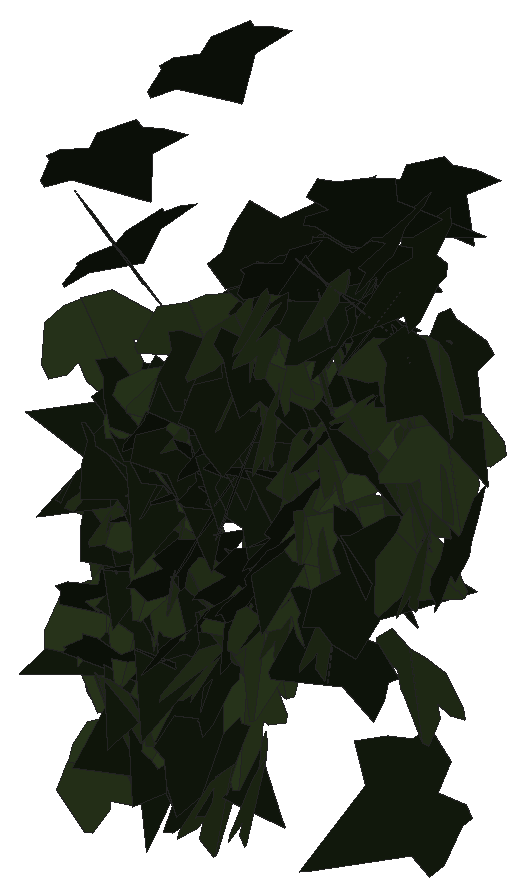
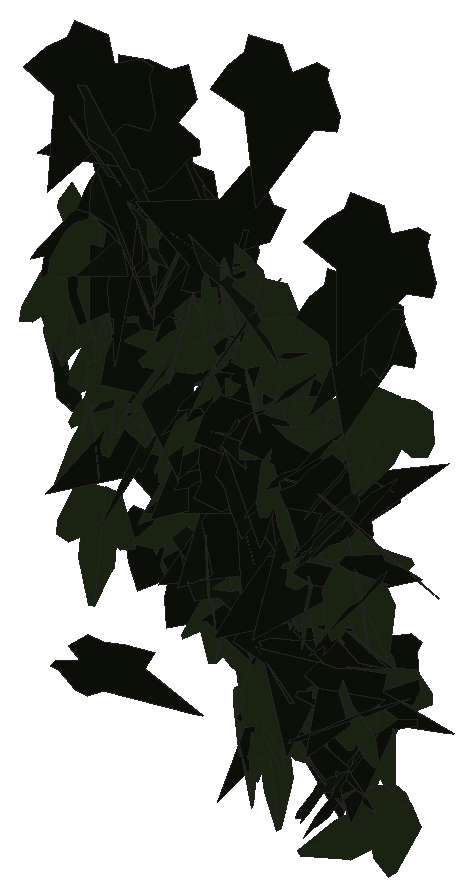
# SketchUp Ruby script. Lengths in inches.
U = 1.inch
M = Sketchup.active_model
def pt(a) = Geom::Point3d.new(a.map { |v| v * U })
def face(e, loops, mat)
  f = e.add_face(loops[0].map { |a| pt(a) })
  loops[1..].each { |l| e.add_face(l.map { |a| pt(a) }).erase! }
  f.material = f.back_material = mat if mat
  f
end
# faces: each face lists its corners as indices into pts; further lists are holes
def faces(e, pts, list, mat = nil) = list.each { |f| face(e, (f[0].is_a?(Array) ? f : [f]).map { |l| l.map { |i| pts[i] } }, mat) }
# xy, xz, yz: faces in a plane at the given z, y or x. An outline is a flat list of corners, or four numbers for a rectangle; further outlines are holes
def ring(l) = l.size == 4 ? [[l[0], l[1]], [l[2], l[1]], [l[2], l[3]], [l[0], l[3]]] : l.each_slice(2).to_a
def flat(e, list, mat, &to3) = list.each { |f| face(e, (f[0].is_a?(Array) ? f : [f]).map { |l| ring(l).map { |u, v| to3.(u, v) } }, mat) }
def xy(e, z, list, mat = nil) = flat(e, list, mat) { |x, y| [x, y, z] }
def xz(e, y, list, mat = nil) = flat(e, list, mat) { |x, z| [x, y, z] }
def yz(e, x, list, mat = nil) = flat(e, list, mat) { |y, z| [x, y, z] }
def lines(e, pts, list) = list.each { |a, b| e.add_line(pt(pts[a]), pt(pts[b])) }
# prism: a flat outline (further loops are holes) pulled along v
def prism(e, loops, v, mat = nil)
  f = face(e, loops, mat); d = Geom::Vector3d.new(v.map { |x| x * U })
  f.pushpull(f.normal.samedirection?(d) ? d.length : -d.length)
end
def box(e, o, s, mat = nil) = prism(e, [[o, [o[0] + s[0], o[1], o[2]], [o[0] + s[0], o[1] + s[1], o[2]], [o[0], o[1] + s[1], o[2]]]], [0, 0, s[2]], mat)
def at(x, y, z, deg = 0) = Geom::Transformation.translation(pt([x, y, z])) * Geom::Transformation.rotation(ORIGIN, Z_AXIS, deg.degrees)
def axes(o, x, y, z) = Geom::Transformation.new([*x, 0, *y, 0, *z, 0, *pt(o).to_a, 1])
def part(name) = M.definitions.add(name)
# library, detail: a bought-in or finely detailed component or shape, given as its bounding box
def library(name, o, s) = part(name).tap { |d| box(d.entities, o, s) }
def detail(e, o, s) = box(e.add_group.entities, o, s)
def put(e, d, t, mat = nil) = e.add_instance(d, t).tap { |i| i.material = mat if mat }
def group(e, t, mat = nil) = e.add_group.tap { |g| g.transformation = t; g.material = mat if mat }.entities
root = M.entities
M.materials.add("efeu1").color = [18, 25, 13]
M.materials.add("efeu2").color = [43, 57, 29]
c1 = part("ivyleaf_10")
p = [[0,0.5,-0.03],[-0.0625,2.02,-0.43],[-0.19,2.01,-0.46],[-0.54,1.05,-0.29],[-0.52,0.625,-0.18],[-0.83,0.76,-0.28],
  [-1.16,0.64,-0.33],[-1.15,0.33,-0.24],[-0.77,-0.39,0.02],[-0.3,-0.51,0.16],[0.04,-0.48,0.23],[-0.02,2.01,-0.4375],
  [-0.06,2.01,-0.43],[0.04,-0.49,0.23],[0.67,-0.49,0.14],[1.38,0.36,-0.2],[1.375,0.51,-0.24],[0.81,0.65,-0.19],
  [0.62,0.59,-0.15],[0.6,1.09,-0.28],[0.5,1.23,-0.31]]
faces(c1.entities,p,[[0,1,2,3,4,5,6,7,8,9,10],[11,12,0,13,14,15,16,17,18,19,20]],"efeu2")
c2 = part("ivyleaf_9")
p = [[1.54,2.16,1.25],[1.36,2.04,1.19],[-0.21,0.99,0.68],[-0.71,1.11,0.82],[-0.85,0.86,0.67],[-0.8,0.17,0.21],
  [-0.9,-0.01,0.1],[-0.67,-0.16,-0.02],[-0.08,-0.08,-0.05],[-0.03,-0.6,-0.4],[0.65,-0.88,-0.66],[0.83,-0.6,-0.49],
  [1.29,-0.42,-0.43],[1.8125,-0.07,-0.26],[1.21,0.44,0.15]]
faces(c2.entities,p,[[0,1,2,3,4,5,6,7,8,9,10,11,12,13,14]],"efeu1")
put(root,c1,axes([35.52,223.96,228.77],[-0.15794,-0.42054,-0.21955],[0.07489,0.20639,-0.44921],[0.46845,-0.17478,-0.0022]))
put(root,c1,axes([35.24,224.09,223.65],[0.05182,-0.4899,-0.0855],[-0.02172,0.08365,-0.49247],[0.49683,0.05475,-0.01262]))
put(root,c2,axes([37,223.73,226.66],[0.10287,0.0619,-0.48537],[-0.07928,0.49154,0.04589],[0.48284,0.06752,0.11094]))
put(root,c1,axes([35.87,224.14,228.92],[0.06062,-0.49536,-0.03074],[0.00028,0.03101,-0.49904],[0.49631,0.06048,0.00404]))
put(root,c1,axes([34.51,224.03,227.63],[0.41045,0.27365,0.08151],[0.02159,0.11258,-0.48668],[-0.28472,0.40304,0.0806]))
put(root,c1,axes([35.71,224.14,229.06],[0.16315,-0.47129,-0.03561],[0.00214,0.03841,-0.49852],[0.47263,0.16252,0.01455]))
put(root,c1,axes([34.15,224.17,225.34],[0.49772,-0.0464,-0.01106],[-0.01119,-0.0008,-0.49987],[0.04637,0.49784,-0.00183]))
put(root,c2,axes([35.02,224.33,227.81],[-0.03439,-0.49861,-0.01448],[0.00897,0.0139,-0.49973],[0.49874,-0.03463,0.00799]))
put(root,c1,axes([37.9,224.14,228.24],[-0.26587,-0.42079,-0.04744],[0.13104,-0.02848,-0.48168],[0.40267,-0.26856,0.12542]))
put(root,c1,axes([33.87,224.05,224.1],[-0.45825,0.19556,-0.04199],[0.03608,-0.02242,-0.49819],[-0.19673,-0.45962,0.00644]))
put(root,c2,axes([34.05,224.23,227.47],[0.25315,-0.43099,0.01288],[0.02635,0.00056,-0.49931],[0.43037,0.25348,0.02299]))
put(root,c1,axes([37.78,224.09,229.05],[0.4487,-0.2169,0.04034],[0.10045,0.11946,-0.47501],[0.19642,0.43438,0.15078]))
put(root,c2,axes([35.21,223.92,223.78],[-0.24544,0.33182,0.28223],[-0.19825,0.20337,-0.41151],[-0.38789,-0.31391,0.03174]))
put(root,c1,axes([37.67,224.04,227.08],[0.19131,-0.42538,-0.18014],[-0.04582,0.17654,-0.46555],[0.45968,0.19463,0.02857]))
put(root,c1,axes([36.54,224.09,226],[0.14851,-0.46443,-0.11067],[0.00063,0.11609,-0.48634],[0.47744,0.14431,0.03506]))
put(root,c2,axes([36.74,224.11,225.74],[0.06549,0.0969,-0.48613],[-0.41934,-0.25065,-0.10645],[-0.26433,0.42165,0.04844]))
put(root,c1,axes([35.8125,224.09,227.92],[0.22839,-0.43074,-0.11089],[0.01971,0.13434,-0.48121],[0.44435,0.21544,0.07835]))
put(root,c2,axes([33.77,223.99,229.26],[0.46569,-0.11467,-0.14136],[-0.13181,0.05537,-0.47913],[0.12554,0.48351,0.02134]))
put(root,c2,axes([36.75,223.875,230.49],[0.38317,0.08091,0.31086],[0.2953,0.10168,-0.39046],[-0.1264,0.48282,0.03014]))
put(root,c2,axes([35.46,223.85,228.18],[0.15851,-0.12531,-0.45735],[-0.07051,0.47064,-0.15339],[0.46894,0.11312,0.13153]))
put(root,c2,axes([34.33,224.38,226.8125],[-0.14137,-0.00782,0.47954],[-0.44716,-0.17859,-0.13473],[0.17339,-0.46695,0.0435]))
put(root,c2,axes([35.56,223.77,226.95],[0.08008,0.07508,0.4878],[0.04245,0.4913,-0.08258],[-0.49172,0.05464,0.07231]))
put(root,c2,axes([35.19,224.24,228.19],[-0.17493,-0.40483,-0.23561],[0.09349,0.21627,-0.44101],[0.45898,-0.19835,0.00003]))
put(root,c2,axes([36.64,224.09,229.3125],[-0.32127,0.28919,0.25131],[-0.27364,0.05635,-0.41466],[-0.26815,-0.40397,0.12206]))
put(root,c2,axes([35.75,224.41,226.88],[-0.10894,-0.4873,0.02594],[-0.00635,-0.02516,-0.49933],[0.48795,-0.10913,-0.00071]))
put(root,c2,axes([37.68,224.18,230.17],[-0.44218,0.23119,-0.0321],[0.02923,-0.01336,-0.49897],[-0.23157,-0.44314,-0.0017]))
put(root,c1,axes([36.25,224.19,229.26],[-0.44111,-0.17762,0.15452],[-0.12742,-0.09582,-0.4739],[0.19796,-0.45746,0.03927]))
put(root,c1,axes([35.34,224.23,228.03],[0.23101,-0.44309,0.0175],[0.00756,-0.0158,-0.49969],[0.44337,0.23113,-0.0006]))
put(root,c2,axes([36.02,224.14,229.07],[0.2194,-0.08043,0.44203],[0.41564,-0.15045,-0.23368],[0.17059,0.47,0.00084]))
put(root,c1,axes([34.9,224.11,228.55],[-0.39357,-0.27685,-0.13587],[0.14092,0.0345,-0.47849],[0.27431,-0.41493,0.05087]))
put(root,c2,axes([34.125,224.54,223.59],[-0.06005,-0.32774,0.3728],[0.07015,-0.37735,-0.32044],[0.4914,0.01382,0.09131]))
put(root,c2,axes([35.14,223.88,231.61],[0.17246,0.4691,0.01434],[0.00467,0.01356,-0.49979],[-0.46929,0.17252,0.0003]))
put(root,c1,axes([34.29,224.23,225.95],[-0.36066,-0.22563,0.26271],[-0.22969,-0.12801,-0.42527],[0.25916,-0.42744,-0.01132]))
put(root,c2,axes([34.5,224.39,227.09],[-0.32415,-0.37301,-0.07607],[0.05769,0.05063,-0.49407],[0.37629,-0.32909,0.01022]))
put(root,c1,axes([35.59,224.13,223.83],[0.19074,-0.44344,-0.13031],[-0.03973,0.12472,-0.48256],[0.46048,0.19444,0.01234]))
put(root,c2,axes([35.52,224.0625,228.62],[0.29268,-0.3076,-0.26405],[-0.1591,0.21238,-0.42377],[0.37286,0.33208,0.02644]))
put(root,c2,axes([36.17,223.875,229.68],[0.31164,0.39051,0.01944],[0.00341,0.02214,-0.4995],[-0.39098,0.31146,0.01113]))
put(root,c2,axes([34.07,223.99,224.62],[0.32074,0.2814,-0.26065],[-0.24394,-0.11256,-0.42169],[-0.29601,0.39767,0.06509]))
put(root,c2,axes([33.95,224.57,223.63],[0.20155,-0.28904,-0.35474],[0.19057,-0.29938,0.35221],[-0.41601,-0.27718,-0.01051]))
put(root,c2,axes([34.23,224.26,226.83],[-0.47418,0.14861,0.05541],[-0.06972,-0.03843,-0.49362],[-0.14246,-0.47585,0.05717]))
put(root,c2,axes([33.8,223.88,230.11],[0.26621,0.42299,0.0144],[0.00483,0.01397,-0.49978],[-0.42321,0.26624,0.00336]))
put(root,c1,axes([34.875,224.16,225.67],[-0.42422,0.13348,-0.22852],[0.21515,-0.07748,-0.44464],[-0.15412,-0.47558,0.0083]))
put(root,c1,axes([33.64,224.03,228.09],[0.36696,0.27323,0.20171],[0.08739,0.21099,-0.4448],[-0.32818,0.3617,0.1071]))
put(root,c1,axes([36.57,224.21,229.46],[0.08804,-0.49081,-0.0368],[-0.00027,0.03734,-0.4986],[0.49219,0.08782,0.00631]))
put(root,c1,axes([34.82,224.24,227.69],[-0.35532,-0.35131,0.01808],[0.05364,-0.0795,-0.49072],[0.34767,-0.34678,0.09418]))
put(root,c2,axes([36.77,224.1,229.31],[-0.34402,0.36065,0.03972],[-0.0341,0.02235,-0.49833],[-0.36123,-0.34559,0.00922]))
put(root,c2,axes([35.45,224.33,228.05],[-0.06953,-0.46957,-0.15707],[0.04009,0.15275,-0.4744],[0.49352,-0.07856,0.01641]))
put(root,c2,axes([37.27,223.98,229.53],[-0.17331,0.46218,0.07969],[-0.01226,0.08046,-0.49333],[-0.46884,-0.17295,-0.01655]))
put(root,c2,axes([35.02,224.02,224.22],[0.13723,-0.27077,-0.3973],[-0.13808,0.37357,-0.30229],[0.46054,0.19269,0.02776]))
put(root,c2,axes([33.99,224.28,226.86],[0.09239,-0.4653,-0.15799],[-0.01471,0.15806,-0.47413],[0.49117,0.09225,0.01552]))
put(root,c2,axes([34.63,224.38,227.22],[0.04884,-0.49538,-0.04705],[-0.00109,0.04717,-0.49777],[0.49761,0.04873,0.00353]))
put(root,c2,axes([37.65,224.19,229.17],[0.12942,-0.41312,-0.25017],[-0.06756,0.24096,-0.43287],[0.47821,0.14584,0.00654]))
put(root,c1,axes([35.68,224.1875,228.48],[0.49581,-0.06398,0.00868],[0.02156,0.10071,-0.48928],[0.06086,0.48556,0.10262]))
put(root,c1,axes([37.56,224.18,227.91],[-0.43961,0.21485,0.10286],[-0.14183,-0.06262,-0.47536],[-0.19138,-0.44712,0.116]))
put(root,c1,axes([35.24,224.46,226.33],[0.06548,-0.06117,0.4919],[0.41809,-0.25974,-0.08796],[0.26629,0.42284,0.01713]))
put(root,c2,axes([35.78,223.8,226.12],[0.13919,0.35786,0.32026],[0.08866,0.30855,-0.38332],[-0.47198,0.1635,0.02244]))
put(root,c1,axes([34.4,224.5,225.96],[-0.12843,0.20564,-0.43729],[0.11586,-0.42617,-0.23443],[-0.46913,-0.16155,0.06181]))
put(root,c1,axes([34.82,224.27,227.46],[0.46548,0.17948,-0.03337],[-0.02644,-0.02414,-0.49872],[-0.18063,0.46605,-0.01298]))
put(root,c2,axes([36.81,224.09,229.92],[0.29238,0.33013,-0.23564],[-0.16206,-0.17121,-0.44094],[-0.37182,0.33422,0.00688]))
put(root,c2,axes([36.06,223.81,226.73],[0.12825,0.32142,0.36089],[0.11646,0.34182,-0.34582],[-0.46903,0.17276,0.01282]))
put(root,c1,axes([37.38,224.22,228.95],[-0.41138,-0.28403,-0.0096],[0.01363,-0.00286,-0.49981],[0.28387,-0.41148,0.0101]))
put(root,c2,axes([34.5,224.49,225.22],[-0.28829,-0.40651,-0.04048],[0.04771,0.01571,-0.49747],[0.40573,-0.29069,0.02973]))
put(root,c1,axes([34.39,224.32,226.09],[0.31111,0.35743,-0.15954],[-0.10617,-0.1191,-0.47386],[-0.37675,0.32872,0.00179]))
put(root,c2,axes([34.05,223.92,229.15],[0.09935,0.4815,0.09101],[-0.03175,0.099,-0.48907],[-0.489,0.0914,0.05025]))
put(root,c2,axes([37.41,224.07,230.44],[-0.25608,0.42072,0.08615],[-0.05093,0.06985,-0.49247],[-0.42642,-0.261,0.00708]))
put(root,c2,axes([35.26,224.45,226.78],[0.20537,0.13041,0.43683],[-0.36358,-0.24218,0.24323],[0.27502,-0.41754,-0.00464]))
put(root,c2,axes([35.28,223.99,226.91],[0.44002,0.07491,0.22532],[0.20948,0.1009,-0.44265],[-0.11178,0.48395,0.05741]))
put(root,c1,axes([33.64,224.25,224.9],[0.39056,0.31161,0.01887],[0.01641,0.00969,-0.49964],[-0.31175,0.3909,-0.00265]))
put(root,c2,axes([34.77,224.03,227.61],[0.06052,0.49508,-0.03511],[-0.00346,-0.03495,-0.49877],[-0.49631,0.06062,-0.00081]))
put(root,c1,axes([36.1,224.09,226.77],[-0.14103,-0.12724,0.46252],[0.36171,0.28845,0.18964],[-0.31508,0.38808,0.01069]))
put(root,c2,axes([35.75,223.97,229.37],[-0.01432,-0.01915,0.49943],[0.42412,0.26387,0.02228],[-0.26442,0.42427,0.00869]))
put(root,c2,axes([35.35,224.39,227.09],[-0.29354,0.27273,-0.29909],[0.17479,-0.24783,-0.39753],[-0.36508,-0.33794,0.05016]))
put(root,c2,axes([34.7,223.89,225.86],[0.31933,0.28911,0.25386],[0.16515,0.19496,-0.42978],[-0.34749,0.35834,0.02902]))
put(root,c2,axes([35.48,223.87,226.07],[0.27867,0.26976,0.31555],[0.17583,0.26758,-0.38404],[-0.37606,0.32501,0.05427]))
put(root,c1,axes([36.29,224.18,228.65],[-0.31011,0.39198,0.01368],[-0.01592,0.00485,-0.49972],[-0.39189,-0.31037,0.00947]))
put(root,c2,axes([36.34,224.18,229.47],[0.45409,-0.1895,0.08886],[0.11402,0.04595,-0.48465],[0.17552,0.46041,0.08494]))
put(root,c2,axes([36.71,224.14,227.02],[0.36115,-0.21409,-0.27155],[-0.2231,0.15573,-0.41949],[0.26419,0.42416,0.01696]))
put(root,c1,axes([35.23,224.35,224.59],[0.48265,-0.0584,0.1168],[0.11441,-0.02646,-0.48601],[0.06294,0.49587,-0.01218]))
put(root,c1,axes([34.26,224.22,226.29],[-0.2162,-0.43719,-0.1101],[0.06292,0.09164,-0.48749],[0.44643,-0.22464,0.01539]))
put(root,c1,axes([36.07,224.35,227.36],[-0.02331,0.46823,-0.17384],[-0.01615,-0.17465,-0.46823],[-0.4992,-0.01621,0.02326]))
put(root,c2,axes([37.3125,224.29,228.89],[0.05269,0.15309,-0.47306],[-0.36654,-0.30947,-0.14098],[-0.33596,0.36165,0.07962]))
put(root,c2,axes([35.9375,224.13,229.24],[-0.2908,0.3727,0.16288],[-0.12579,0.108,-0.47171],[-0.3868,-0.31532,0.03096]))
put(root,c2,axes([35.4,224.07,227.53],[0.02404,0.49767,-0.04175],[0.00736,-0.04215,-0.49817],[-0.49937,0.02334,-0.00936]))
put(root,c1,axes([35.78,224.13,228.4],[-0.19572,-0.13064,-0.44117],[0.41874,0.1481,-0.22962],[0.19067,-0.45935,0.05143]))
put(root,c2,axes([36.54,224.29,227.9],[0.37195,-0.33348,-0.02116],[0.01253,0.04556,-0.49776],[0.33392,0.36975,0.04225]))
put(root,c1,axes([37.48,224.2,225.64],[-0.48026,0.09318,0.10329],[-0.10049,0.02434,-0.48919],[-0.09619,-0.49064,-0.00465]))
put(root,c1,axes([37.28,224.22,227.52],[-0.48712,0.08177,0.07765],[-0.07947,-0.00463,-0.49362],[-0.08001,-0.49325,0.0175]))
put(root,c1,axes([35.55,224.375,225.46],[0.09822,0.45803,-0.17481],[-0.03142,-0.17204,-0.46842],[-0.48925,0.103,-0.00501]))
put(root,c2,axes([34.76,224.16,225.3125],[-0.23421,0.16416,0.41012],[-0.31713,0.26067,-0.28545],[-0.30752,-0.39383,-0.01798]))
put(root,c1,axes([33.8125,224.45,226.1875],[-0.09706,-0.46045,0.169],[-0.01219,-0.16996,-0.47007],[0.49034,-0.09537,0.02177]))
put(root,c2,axes([33.92,224.31,227.125],[0.33961,-0.36595,-0.0274],[0.04425,0.07789,-0.49191],[0.36429,0.33169,0.08529]))
put(root,c2,axes([33.99,224.52,226.29],[-0.29996,-0.38614,-0.1045],[0.08617,0.06518,-0.48819],[0.39064,-0.31088,0.02744]))
put(root,c2,axes([35.06,224.32,224.78],[-0.4323,0.24491,-0.05603],[0.05129,-0.02312,-0.49682],[-0.24595,-0.4353,-0.00514]))
put(root,c2,axes([34.1,224.32,226.9],[0.34619,-0.36076,-0.00262],[0.05679,0.05809,-0.49336],[0.35627,0.34129,0.08119]))
put(root,c1,axes([35.59,224.31,228.27],[-0.08482,0.48319,-0.09663],[0.00044,-0.09797,-0.49031],[-0.49275,-0.08326,0.01619]))
put(root,c2,axes([33.8,224.03,225.28],[0.38419,0.31983,0.01038],[0.00774,0.00692,-0.49989],[-0.31991,0.38426,0.00036]))
put(root,c2,axes([37.46,224.04,230.97],[0.34187,0.36478,-0.00771],[-0.0043,-0.00654,-0.49994],[-0.36484,0.3419,-0.00134]))
put(root,c2,axes([38.09,223.96,227.01],[0.03261,0.15554,0.47407],[-0.09281,0.46868,-0.14739],[-0.49023,-0.07839,0.05944]))
put(root,c2,axes([33.75,224.43,225.94],[0.16189,-0.46609,-0.08095],[-0.03348,0.07405,-0.49335],[0.47188,0.16516,-0.00724]))
put(root,c2,axes([35.1,224.1,227.06],[0.38981,0.23179,-0.21053],[-0.22056,-0.03537,-0.44733],[-0.22227,0.44161,0.07468]))
put(root,c1,axes([37.41,224.14,226.97],[-0.01897,-0.39782,-0.3023],[0.19094,0.27378,-0.37227],[0.46172,-0.12957,0.14153]))
put(root,c1,axes([36.4,224.23,229.13],[-0.25107,0.4312,0.03212],[-0.01092,0.03081,-0.49893],[-0.43226,-0.25123,-0.00605]))
put(root,c2,axes([35.72,224.35,225.72],[0.01761,0.38213,-0.32197],[-0.06972,-0.31714,-0.38021],[-0.4948,0.05829,0.04211]))
put(root,c2,axes([34.1,224.5625,224.8],[-0.42672,-0.09443,0.24288],[-0.23482,-0.06272,-0.43695],[0.11299,-0.48698,0.00918]))
put(root,c1,axes([36.41,224.27,226.48],[-0.14345,0.47894,-0.00589],[-0.00242,-0.00688,-0.49995],[-0.47897,-0.14341,0.00429]))
put(root,c2,axes([35.87,224.33,225.84],[-0.29594,0.38937,-0.10397],[-0.00063,-0.12944,-0.48296],[-0.40301,-0.28572,0.07711]))
put(root,c1,axes([35.5625,224.37,225.56],[-0.40279,-0.28988,-0.06105],[0.10778,-0.04742,-0.48594],[0.27594,-0.40462,0.10068]))
put(root,c1,axes([33.8,224.39,226.39],[0.25397,-0.43001,-0.02429],[0.02573,0.0433,-0.49746],[0.42992,0.25143,0.04413]))
put(root,c2,axes([34.26,224.52,224],[-0.37076,-0.12049,-0.31308],[0.31564,0.03275,-0.38639],[0.11362,-0.48416,0.05178]))
put(root,c1,axes([33.61,224.11,223.25],[-0.07907,-0.17664,-0.46102],[0.37224,0.28538,-0.17319],[0.32432,-0.37061,0.08637]))
put(root,c1,axes([36.47,224.27,227.75],[-0.0814,0.49268,0.0252],[0.00019,0.02558,-0.49935],[-0.49333,-0.08129,-0.00435]))
put(root,c2,axes([37.35,224.59,224.02],[-0.44596,-0.1414,0.17643],[-0.17114,-0.04389,-0.46775],[0.14776,-0.47758,-0.00925]))
put(root,c1,axes([34.5625,224.5,224.3125],[0.28514,0.32115,-0.25604],[-0.17408,-0.18782,-0.42944],[-0.37201,0.33404,0.00471]))
put(root,c1,axes([36.71,224.23,227.98],[-0.25487,-0.36618,-0.22573],[0.11476,0.19499,-0.44588],[0.41457,-0.2791,-0.01535]))
put(root,c1,axes([35.79,224.36,225.76],[0.18388,-0.45298,-0.10487],[0.00112,0.11321,-0.48701],[0.46496,0.17887,0.04265]))
put(root,c1,axes([36.83,224.54,227.85],[0.30788,0.2465,-0.30732],[-0.23305,-0.20051,-0.39431],[-0.31764,0.38605,-0.00857]))
put(root,c1,axes([37.48,224.13,227.76],[-0.25839,0.29879,0.30653],[-0.19485,0.2367,-0.39498],[-0.38114,-0.32357,-0.00588]))
put(root,c2,axes([37.15,224.22,229.21],[0.26311,0.0037,-0.42516],[-0.42388,0.04128,-0.26196],[0.03316,0.49828,0.02486]))
put(root,c2,axes([36.66,224.24,227.99],[-0.05415,0.49084,-0.07839],[0.00024,-0.07883,-0.49375],[-0.49706,-0.05351,0.0083]))
put(root,c2,axes([33.89,224.77,224.52],[-0.22415,-0.42927,0.12446],[0.08945,-0.1795,-0.45802],[0.4379,-0.18306,0.15726]))
put(root,c1,axes([34.75,224.43,227.22],[-0.03827,-0.49733,-0.03457],[-0.00945,0.03539,-0.49866],[0.49844,-0.03751,-0.0121]))
put(root,c1,axes([36.04,224.32,226.09],[0.18191,0.45858,0.0813],[0.01327,0.08214,-0.49303],[-0.46555,0.18153,0.01772]))
put(root,c2,axes([34.41,224.0625,226.32],[0.31953,0.35726,0.14237],[0.01857,0.17054,-0.46965],[-0.38413,0.30542,0.09571]))
put(root,c2,axes([34.8,224.16,225.12],[0.02652,0.49275,0.08059],[-0.01473,0.08144,-0.4931],[-0.49908,0.02378,0.01883]))
put(root,c1,axes([33.75,224.57,224.66],[0.35352,-0.08843,0.34235],[0.33397,-0.0755,-0.36436],[0.11613,0.48629,0.00569]))
put(root,c1,axes([34.86,224.5,224.67],[-0.07114,-0.49491,0.00074],[0.01234,-0.00252,-0.49984],[0.49476,-0.0711,0.01257]))
